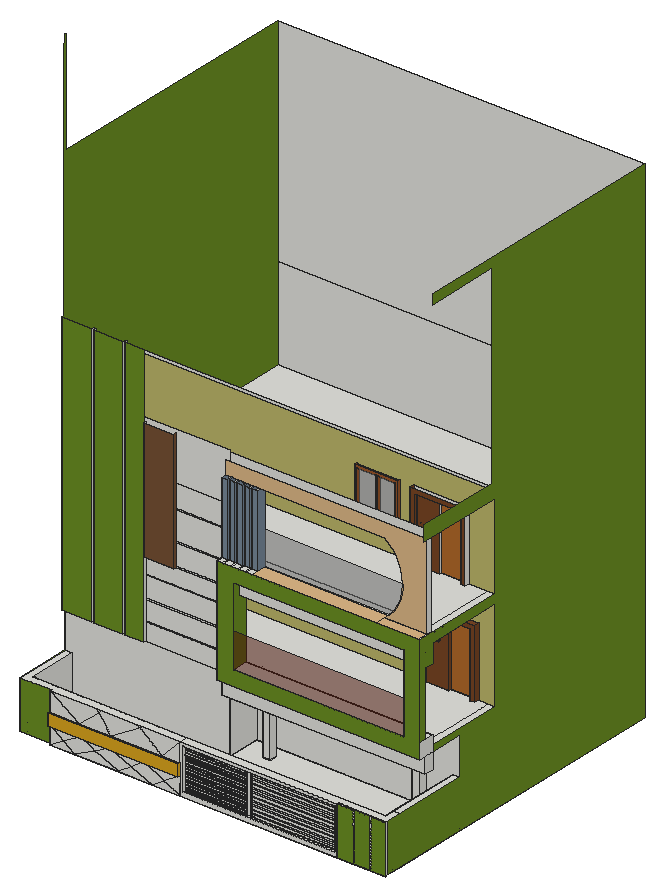
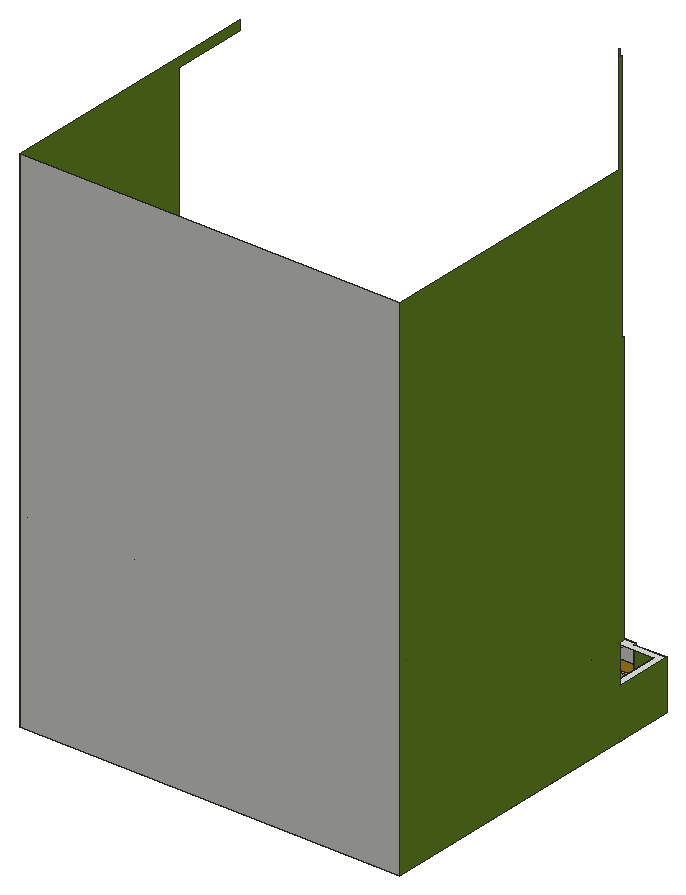
# SketchUp Ruby script. Lengths in inches.
U = 1.inch
M = Sketchup.active_model
def pt(a) = Geom::Point3d.new(a.map { |v| v * U })
def face(e, loops, mat)
  f = e.add_face(loops[0].map { |a| pt(a) })
  loops[1..].each { |l| e.add_face(l.map { |a| pt(a) }).erase! }
  f.material = f.back_material = mat if mat
  f
end
# faces: each face lists its corners as indices into pts; further lists are holes
def faces(e, pts, list, mat = nil) = list.each { |f| face(e, (f[0].is_a?(Array) ? f : [f]).map { |l| l.map { |i| pts[i] } }, mat) }
# xy, xz, yz: faces in a plane at the given z, y or x. An outline is a flat list of corners, or four numbers for a rectangle; further outlines are holes
def ring(l) = l.size == 4 ? [[l[0], l[1]], [l[2], l[1]], [l[2], l[3]], [l[0], l[3]]] : l.each_slice(2).to_a
def flat(e, list, mat, &to3) = list.each { |f| face(e, (f[0].is_a?(Array) ? f : [f]).map { |l| ring(l).map { |u, v| to3.(u, v) } }, mat) }
def xy(e, z, list, mat = nil) = flat(e, list, mat) { |x, y| [x, y, z] }
def xz(e, y, list, mat = nil) = flat(e, list, mat) { |x, z| [x, y, z] }
def yz(e, x, list, mat = nil) = flat(e, list, mat) { |y, z| [x, y, z] }
def lines(e, pts, list) = list.each { |a, b| e.add_line(pt(pts[a]), pt(pts[b])) }
# prism: a flat outline (further loops are holes) pulled along v
def prism(e, loops, v, mat = nil)
  f = face(e, loops, mat); d = Geom::Vector3d.new(v.map { |x| x * U })
  f.pushpull(f.normal.samedirection?(d) ? d.length : -d.length)
end
def box(e, o, s, mat = nil) = prism(e, [[o, [o[0] + s[0], o[1], o[2]], [o[0] + s[0], o[1] + s[1], o[2]], [o[0], o[1] + s[1], o[2]]]], [0, 0, s[2]], mat)
def at(x, y, z, deg = 0) = Geom::Transformation.translation(pt([x, y, z])) * Geom::Transformation.rotation(ORIGIN, Z_AXIS, deg.degrees)
def axes(o, x, y, z) = Geom::Transformation.new([*x, 0, *y, 0, *z, 0, *pt(o).to_a, 1])
def part(name) = M.definitions.add(name)
# library, detail: a bought-in or finely detailed component or shape, given as its bounding box
def library(name, o, s) = part(name).tap { |d| box(d.entities, o, s) }
def detail(e, o, s) = box(e.add_group.entities, o, s)
def put(e, d, t, mat = nil) = e.add_instance(d, t).tap { |i| i.material = mat if mat }
def group(e, t, mat = nil) = e.add_group.tap { |g| g.transformation = t; g.material = mat if mat }.entities
root = M.entities
M.materials.add("[0036_BurlyWood]").color = [222, 184, 135]
M.materials.add("[0045_Goldenrod]").color = [218, 165, 32]
M.materials.add("[0057_DarkKhaki]").color = [189, 183, 107]
M.materials.add("[0061_OliveDrab]").color = [107, 142, 35]
M.materials.add("[0110_LightSlateGray]").color = [119, 136, 153]
M.materials.add("[Sandstone]").color = [118, 81, 52]
M.materials.add("[Translucent Glass Dark Green]").color = [91, 24, 11]
M.materials["[Translucent Glass Dark Green]"].alpha = 0.5
M.materials.add("[Translucent Glass Gray]").color = [128, 128, 128]
M.materials["[Translucent Glass Gray]"].alpha = 0.5
M.materials.add("[Wood Bamboo]").color = [177, 105, 43]
M.materials.add("[Wood Cherry Original]").color = [152, 86, 42]
M.materials.add("[Wood Veneer 01]").color = [120, 70, 37]
xy(root,0,[[[211.33,3,417,3,417,6,480,6,480,15,471,15,471,123.9375,214.69,123.9375,214.69,79.75,9,79.75,9,15,211.33,15],[242.41,99.05,252.1,108.74],[438.16,99.05,447.85,108.74]],[40.99,3,211.33,6],[417,3,480,6],[0,6,9,15],[0,15,9,79.75],
  [471,15,480,26.9375],[471,26.9375,480,123.9375],[0,79.75,9,81.3125],[9,79.75,214.69,81.3125],[0,81.3125,9,88.75],
  [9,81.3125,9,88.75,205.69,88.75,205.69,123.9375,214.69,123.9375,214.69,81.3125],[0,88.75,9,123.9375],[9,88.75,205.69,123.9375],[242.41,99.05,252.1,108.74],[438.16,99.05,447.85,108.74],
  [0,123.9375,205.69,123.9375,205.69,132.9375,480,132.9375,480,426.3125,0,426.3125],[205.69,123.9375,205.69,129.9375,471,129.9375,471,132.9375,480,132.9375,480,123.9375],[205.69,129.9375,471,132.9375]])
xy(root,3,[[[9,15,471,15,471,123.9375,214.69,123.9375,214.69,79.75,9,79.75],[242.41,99.05,252.1,108.74],[438.16,99.05,447.85,108.74]]])
xy(root,6.12,[[215.375,3,414.15,3,414.15,6,302.66,6,302.66,15,300.97,15,300.97,6,215.375,6]])
xy(root,13.75,[[9,14.75,211.33,15],[211.33,14.75,295.89,15],[295.89,14.75,300.97,15],[302.66,14.75,471,15],[[9,15,471,15,471,123.9375,214.69,123.9375,214.69,79.75,9,79.75],[242.41,99.05,252.1,108.74],[438.16,99.05,447.85,108.74]]])
xy(root,23.125,[[40.99,0,211.33,3]],"[0045_Goldenrod]")
xy(root,38.15,[[40.99,0,211.33,3]])
xy(root,42.09,[[215.375,6,295.89,35.9375]])
xy(root,44.04,[[215.375,6,295.89,35.9375]])
xy(root,45.22,[[215.375,6,295.89,28.75]])
xy(root,47.16,[[215.375,6,295.89,28.75]])
xy(root,48.34,[[215.375,6,295.89,15]])
xy(root,50.29,[[215.375,6,295.89,15]])
xy(root,51.47,[[215.375,6,295.89,15]])
xy(root,53.41,[[215.375,6,295.89,15]])
xy(root,54.59,[[215.375,6,295.89,14.75],[215.375,14.75,295.89,15]])
xy(root,56.54,[[215.375,6,295.89,14.75],[215.375,14.75,295.89,15]])
xy(root,57.72,[[215.375,6,295.89,14.75],[215.375,14.75,295.89,15]])
xy(root,59.66,[[215.375,3,215.375,6,300.97,6,300.97,14.75,302.66,14.75,302.66,6,414.15,6,414.15,3],[215.375,6,295.89,14.75],[215.375,14.75,295.89,15],[300.97,14.75,302.66,15]])
xy(root,63,[[40.99,3,211.33,3,211.33,14.75,9,14.75,9,79.75,0,79.75,0,6,40.99,6],[211.33,3,417,3,417,6,480,6,480,26.9375,471,26.9375,471,15,211.33,15],[417,3,480,6],[9,14.75,211.33,15],[471,26.9375,480,123.9375]])
xy(root,91.22,[[214.69,67.75,480,79.75]])
xy(root,108.375,[[438.16,97.62,447.85,99.05],[438.16,99.05,447.85,108.74]])
xy(root,111.625,[[9,81.3125,214.69,123.9375]])
xy(root,112.1,[[0,73.75,0,79.75,214.69,79.75,214.69,76.75,107.35,76.75,107.35,73.75,83.22,73.75,83.22,76.75,80.57,76.75,80.57,73.75,42.34,73.75,42.34,76.75,39.7,76.75,39.7,73.75],[242.41,99.05,252.1,108.74],[252.1,99.05,253.72,108.74]])
xy(root,112.1,[[214.69,58.75,480,67.75]],"[0061_OliveDrab]")
xy(root,120,[[214.69,79.75,480,79.75,480,182.4375,471,182.4375,471,88.75,9,88.75,9,81.3125,214.69,81.3125],[9,79.75,214.69,81.3125],[9,88.75,471,88.75,471,182.4375,458.11,182.4375,458.11,176.4375,452.11,176.4375,452.11,182.4375,422.11,182.4375,422.11,179.4375,392.11,179.4375,392.11,176.4375,386.11,176.4375,386.11,182.4375,9,182.4375],[386.11,176.4375,392.11,182.4375],[452.11,176.4375,458.11,182.4375],
  [392.11,179.4375,422.11,182.4375],[9,188.4375,471,417.3125]])
xy(root,132.05,[[236.55,58.75,459.14,58.75,459.14,67.75,480,67.75,480,79.75,236.55,79.75]])
xy(root,144.9,[[283.375,179.4375,362.5625,182.4375]])
xy(root,147.9,[[286.375,179.4375,322.97,182.4375],[327.14,179.4375,359.5625,182.4375]],"[Wood Cherry Original]")
xy(root,173.57,[[395.1,177.4375,395.1,179.4375,398.85,179.4375,398.85,178.4375,405.85,178.4375,405.85,179.4375,409.6,179.4375,409.6,177.4375]],"[Wood Veneer 01]")
xy(root,174.88,[[395.1,177.4375,409.6,177.4375,409.6,179.4375,405.85,179.4375,405.85,178.4375,398.85,178.4375,398.85,179.4375,395.1,179.4375]],"[Wood Veneer 01]")
xy(root,204,[[392.11,176.4375,392.11,179.4375,422.11,179.4375,422.11,182.4375,452.11,182.4375,452.11,176.4375],[392.11,179.4375,422.11,182.4375]])
xy(root,207.33,[[286.375,179.4375,322.97,182.4375],[327.14,179.4375,359.5625,182.4375]],"[Wood Cherry Original]")
xy(root,210,[[386.11,176.4375,458.11,182.4375]],"[Wood Veneer 01]")
xy(root,210.33,[[283.375,179.4375,362.5625,182.4375]])
xy(root,212.44,[[107.35,73.75,146.78,76.75]],"[Sandstone]")
xy(root,215.25,[[236.55,67.75,480,79.75]])
xy(root,233.625,[[236.55,58.75,459.14,67.75]],"[0061_OliveDrab]")
xy(root,240,[[9,79.75,214.69,81.3125],[479.5625,79.75,480,83.125],[479.5625,83.125,480,182.4375],[9,182.4375,471,188.4375],[8.5625,188.4375,9,192.0625],
  [9,188.4375,336.04,192.0625],[336.04,188.4375,471,192.0625],[336.04,192.0625,471,417.3125]])
xy(root,240,[[214.69,79.75,214.69,81.3125,9,81.3125,9,182.4375,479.5625,182.4375,479.5625,79.75]],"[0057_DarkKhaki]")
xy(root,252,[[214.69,58.75,222.11,67.75],[222.11,58.75,224.38,79.75],[224.38,58.75,231.79,67.75],[231.79,58.75,234.07,79.75],[234.07,58.75,241.48,67.75],
  [241.48,58.75,243.75,79.75],[243.75,58.75,251.17,67.75],[251.17,58.75,253.44,79.75],[253.44,58.75,260.86,67.75],[477.8125,58.75,480,79.75],
  [214.69,67.75,222.11,79.75],[224.38,67.75,231.79,79.75],[234.07,67.75,241.48,79.75],[243.75,67.75,251.17,79.75],[253.44,67.75,260.86,79.75],
  [422.69,73.75,477.8125,79.75],[214.69,79.75,480,79.75,480,182.4375,471,182.4375,471,88.75,9,88.75,9,81.3125,214.69,81.3125],[9,79.75,214.69,81.3125],[9,88.75,471,88.75,471,182.4375,445.35,182.4375,445.35,176.4375,439.35,176.4375,439.35,182.4375,409.35,182.4375,409.35,179.4375,379.35,179.4375,379.35,176.4375,373.35,176.4375,373.35,182.4375,9,182.4375],[373.35,176.4375,379.35,182.4375],
  [439.35,176.4375,445.35,182.4375],[379.35,179.4375,409.35,182.4375],[9,188.4375,471,417.3125]])
xy(root,252,[[260.86,58.75,422.69,79.75],[422.69,58.75,477.8125,73.75]],"[0036_BurlyWood]")
xy(root,289.14,[[298.39,179.4375,354.57,182.4375]],"[Wood Cherry Original]")
xy(root,292.14,[[301.39,179.4375,326.48,182.4375],[329.2,179.4375,351.57,182.4375]],"[Wood Cherry Original]")
xz(root,0,[[40.99,23.125,211.33,38.15]],"[0045_Goldenrod]")
xz(root,3,[[40.99,0,58.6,10.14,40.99,23.125],[40.99,0,72.35,0,58.6,10.14],[72.35,0,100.12,14.13,81.16,23.125,58.6,10.14],[72.35,0,129.9,0,100.12,14.13],[129.9,0,146.75,11.24,117.79,23.125,100.12,14.13],
  [129.9,0,174.13,0,146.75,11.24],[174.13,0,190.61,10.24,164.56,23.125,146.75,11.24],[174.13,0,211.33,0,190.61,10.24],[211.33,0,211.33,23.125,190.61,10.24],[[211.33,0,417,63],[215.375,6.12,414.15,59.66]],
  [436.76,0,438.58,63],[459.14,0,460.95,63],[58.6,10.14,81.16,23.125,40.99,23.125],[190.61,10.24,211.33,23.125,164.56,23.125],[146.75,11.24,164.56,23.125,117.79,23.125],
  [100.12,14.13,117.79,23.125,81.16,23.125],[40.99,38.15,79.4,38.15,40.99,63],[79.4,38.15,104.86,59.64,102.28,63,40.99,63],[79.4,38.15,121.4,38.15,104.86,59.64],[121.4,38.15,158.25,60.54,155.04,63,108.85,63,104.86,59.64],
  [121.4,38.15,187.45,38.15,158.25,60.54],[187.45,38.15,211.33,63,162.29,63,158.25,60.54],[187.45,38.15,211.33,38.15,211.33,63],[104.86,59.64,108.85,63,102.28,63],[158.25,60.54,162.29,63,155.04,63]])
xz(root,3,[[417,0,436.76,63],[438.58,0,459.14,63],[460.95,0,480,63]],"[0061_OliveDrab]")
xz(root,6,[[40.99,0,211.33,3],[417,0,480,63],[302.66,0.71,414.15,3.97],[215.375,1.47,295.89,3.41],[40.99,3,211.33,13.75],
  [215.375,4.59,295.89,6.12],[302.66,5.77,414.15,6.12],[215.375,6.12,295.89,6.54],[295.89,6.12,300.97,59.66],[302.66,6.12,414.15,9.04],
  [215.375,6.54,295.89,7.72],[215.375,7.72,295.89,9.66],[302.66,9.04,414.15,10.84],[215.375,9.66,295.89,10.84],[215.375,10.84,295.89,12.79],
  [302.66,10.84,414.15,14.1],[215.375,12.79,295.89,13.97],[215.375,13.97,295.89,15.91],[302.66,14.1,414.15,15.9],[302.66,15.9,414.15,19.16],
  [215.375,15.91,295.89,17.09],[215.375,17.09,295.89,19.04],[215.375,19.04,295.89,20.22],[302.66,19.16,414.15,20.96],[215.375,20.22,295.89,22.16],
  [302.66,20.96,414.15,24.22],[215.375,22.16,295.89,23.34],[215.375,23.34,295.89,25.29],[302.66,24.22,414.15,26.02],[215.375,25.29,295.89,26.47],
  [302.66,26.02,414.15,29.29],[215.375,26.47,295.89,28.41],[215.375,28.41,295.89,29.59],[302.66,29.29,414.15,31.09],[215.375,29.59,295.89,31.54],
  [302.66,31.09,414.15,34.35],[215.375,31.54,295.89,32.72],[215.375,32.72,295.89,34.66],[302.66,34.35,414.15,36.15],[215.375,34.66,295.89,35.84],
  [215.375,35.84,295.89,37.79],[302.66,36.15,414.15,39.41],[215.375,37.79,295.89,38.97],[215.375,38.97,295.89,40.91],[302.66,39.41,414.15,41.21],
  [215.375,40.91,295.89,42.09],[302.66,41.21,414.15,44.47],[215.375,42.09,295.89,44.04],[215.375,44.04,295.89,45.22],[302.66,44.47,414.15,46.27],
  [215.375,45.22,295.89,47.16],[302.66,46.27,414.15,49.54],[215.375,47.16,295.89,48.34],[215.375,48.34,295.89,50.29],[302.66,49.54,414.15,51.34],
  [215.375,50.29,295.89,51.47],[302.66,51.34,414.15,54.6],[215.375,51.47,295.89,53.41],[215.375,53.41,295.89,54.59],[215.375,54.59,295.89,56.54],
  [302.66,54.6,414.15,56.4],[302.66,56.4,414.15,59.66],[215.375,56.54,295.89,57.72],[215.375,57.72,295.89,59.66]])
xz(root,6,[[0,0,40.99,63]],"[0061_OliveDrab]")
xz(root,15,[[9,3,9,13.75,300.97,13.75,300.97,6.12,302.66,6.12,302.66,13.75,471,13.75,471,3],[300.97,6.12,302.66,13.75]])
xz(root,28.75,[[215.375,45.22,295.89,47.16]])
xz(root,35.9375,[[215.375,42.09,295.89,44.04]])
xz(root,58.75,[[214.69,112.1,480,112.1,480,132.05,236.55,132.05,236.55,233.625,459.14,233.625,459.14,132.05,480,132.05,480,252,214.69,252]],"[0061_OliveDrab]")
xz(root,58.75,[[236.55,132.05,459.14,177.7]],"[Translucent Glass Dark Green]")
xz(root,67.75,[[214.69,91.22,480,112.1],[459.14,132.05,480,215.25],[236.55,215.25,459.14,233.625]])
xz(root,67.75,[[214.69,252,222.11,345.55],[224.38,252,231.79,345.55],[234.07,252,241.48,345.55],[243.75,252,251.17,345.55],[253.44,252,260.86,345.55]],"[0110_LightSlateGray]")
xz(root,73.75,[[422.69,252,477.8125,252,477.8125,363.8125,214.69,363.8125,214.69,345.55,422.69,345.55,429.47,339.59,435.25,332.66,439.9,324.92,443.3,316.56,445.37,307.78,446.07,298.78,445.37,289.78,443.3,280.99,439.9,272.63,435.25,264.89,429.47,257.96]],"[0036_BurlyWood]")
xz(root,73.75,[[0,112.1,39.7,455],[42.34,112.1,80.57,455],[83.22,112.1,107.35,455]],"[0061_OliveDrab]")
xz(root,73.75,[[107.35,212.44,146.78,369.44]],"[Sandstone]")
xz(root,76.75,[[39.7,112.1,42.34,455],[80.57,112.1,83.22,455],[107.35,112.1,214.69,134.76],[107.35,134.76,214.69,136.29],[107.35,136.29,214.69,161.07],
  [107.35,161.07,214.69,162.61],[107.35,162.61,214.69,190.01],[107.35,190.01,214.69,191.54],[107.35,191.54,214.69,191.54,214.69,212.26,146.78,212.26,146.78,212.44,107.35,212.44],[146.78,212.26,214.69,214.11],
  [107.35,212.44,146.78,366.59],[146.78,214.11,214.69,241.33],[146.78,241.33,214.69,243.18],[146.78,243.18,214.69,279.89],[146.78,279.89,214.69,281.74],
  [146.78,281.74,214.69,310.89]])
xz(root,79.75,[[9,0,214.69,3],[9,3,214.69,13.75],[9,13.75,214.69,13.75,214.69,112.1,0,112.1,0,63,9,63],[214.69,91.22,480,112.1],[214.69,112.1,480,120],
  [9,120,214.69,240],[214.69,120,214.69,215.25,236.55,215.25,236.55,132.05,480,132.05,480,120],[214.69,215.25,480,240],[9,252,214.69,372],[446.07,252,446.07,296.15,445.86,296.15,446.07,298.78,445.37,307.78,443.3,316.56,439.9,324.92,435.25,332.66,429.47,339.59,422.69,345.55,214.69,345.55,214.69,370.625,477.8125,370.625,477.8125,252],
  [422.69,252,429.47,257.96,435.25,264.89,439.9,272.63,443.3,280.99,445.37,289.78,445.86,296.15,446.07,296.15,446.07,252]])
xz(root,79.75,[[214.69,252,222.11,296.15],[222.11,252,224.38,296.15],[224.38,252,231.79,296.15],[231.79,252,234.07,296.15],[234.07,252,241.48,296.15],
  [241.48,252,243.75,296.15],[243.75,252,251.17,296.15],[251.17,252,253.44,296.15],[253.44,252,260.86,296.15],[260.86,252,260.86,296.15,445.86,296.15,445.37,289.78,443.3,280.99,439.9,272.63,435.25,264.89,429.47,257.96,422.69,252]],"[Translucent Glass Gray]")
xz(root,81.3125,[[9,0,214.69,111.625],[9,111.625,214.69,112.1]])
xz(root,99.05,[[242.41,0,252.1,3],[438.16,0,447.85,3],[242.41,3,252.1,13.75],[438.16,3,447.85,13.75],[242.41,13.75,252.1,112.1],
  [438.16,13.75,447.85,108.375]])
xz(root,108.74,[[242.41,0,252.1,3],[438.16,0,447.85,3],[242.41,3,252.1,13.75],[438.16,3,447.85,13.75],[242.41,13.75,252.1,112.1],
  [438.16,13.75,447.85,77.75],[438.16,77.75,447.85,108.375]])
xz(root,123.9375,[[9,0,214.69,111.625],[214.69,0,471,3],[214.69,3,471,13.75],[214.69,13.75,471,13.75,471,63,480,63,480,112.1,9,112.1,9,111.625,214.69,111.625]])
xz(root,176.4375,[[386.11,120,392.11,120,392.11,204,452.11,204,452.11,120,458.11,120,458.11,210,386.11,210],[373.35,252,379.35,252,379.35,336,439.35,336,439.35,252,445.35,252,445.35,342,373.35,342]],"[Wood Veneer 01]")
xz(root,177.4375,[[395.1,173.57,409.6,174.88]],"[Wood Veneer 01]")
xz(root,178.4375,[[398.85,173.57,405.85,174.88]])
xz(root,179.4375,[[[283.375,144.9,362.5625,210.33],[286.375,147.9,322.97,207.33],[327.14,147.9,359.5625,207.33]],[[298.39,289.14,354.57,341.33],[301.39,292.14,326.48,338.33],[329.2,292.14,351.57,338.33]]],"[Wood Cherry Original]")
xz(root,179.4375,[[[392.11,120,422.11,204],[395.1,173.57,398.85,174.88],[405.85,173.57,409.6,174.88]],[[379.35,252,409.35,336],[383.79,302.01,386.62,303.76],[395.22,302.01,398.06,303.76]]],"[Wood Veneer 01]")
xz(root,182.4375,[[386.11,114,458.11,120],[392.11,120,422.11,204],[[283.375,144.9,362.5625,210.33],[286.375,147.9,322.97,207.33],[327.14,147.9,359.5625,207.33]],[373.35,246,445.35,252],[373.35,252,373.35,342,445.35,342,445.35,252,439.35,252,439.35,336,379.35,336,379.35,252],
  [379.35,252,409.35,336],[[298.39,289.14,354.57,341.33],[301.39,292.14,326.48,338.33],[329.2,292.14,351.57,338.33]]])
xz(root,182.4375,[[[9,120,386.11,120,386.11,210,458.11,210,458.11,120,480,120,480,240,9,240],[283.375,144.9,362.5625,210.33]],[[9,252,373.35,252,373.35,342,445.35,342,445.35,252,480,252,480,363.8125,477.8125,363.8125,477.8125,372,9,372],[298.39,289.14,354.57,341.33]]],"[0057_DarkKhaki]")
xz(root,182.4375,[[286.375,147.9,322.97,207.33],[327.14,147.9,359.5625,207.33],[301.39,292.14,326.48,338.33],[329.2,292.14,351.57,338.33]],"[Translucent Glass Gray]")
xz(root,182.4375,[[422.11,120,452.11,204],[409.35,252,439.35,336]],"[Wood Bamboo]")
xz(root,188.4375,[[9,120,471,240],[9,252,471,372]])
xz(root,417.3125,[[9,120,471,240],[9,252,471,372]])
xz(root,426.3125,[[0,0,480,648]])
yz(root,0,[[6,0,6,63,79.75,63,79.75,112.1,73.75,112.1,73.75,455,76.75,455,76.75,774.38,79.75,774.38,79.75,784.0625,81.3125,784.0625,81.3125,648,426.3125,648,426.3125,0]],"[0061_OliveDrab]")
yz(root,9,[[15,0,79.75,3],[81.3125,0,123.9375,111.625],[15,3,79.75,3.75],[15,3.75,79.75,3.9375],[15,3.9375,79.75,13.75],
  [14.75,13.75,15,63],[15,13.75,79.75,63],[81.3125,111.625,123.9375,112.5],[79.75,120,81.3125,240],[81.3125,120,88.75,240],
  [88.75,120,182.4375,240],[188.4375,120,417.3125,240],[79.75,252,81.3125,372],[81.3125,252,88.75,372],[88.75,252,182.4375,372]])
yz(root,39.7,[[73.75,112.1,76.75,455]])
yz(root,40.99,[[3,0,3,23.125,0,23.125,0,38.15,3,38.15,3,63,6,63,6,0]],"[0045_Goldenrod]")
yz(root,42.34,[[73.75,112.1,76.75,455]])
yz(root,80.57,[[73.75,112.1,76.75,455]])
yz(root,83.22,[[73.75,112.1,76.75,455]])
yz(root,107.35,[[73.75,112.1,76.75,212.44],[73.75,212.44,76.75,369.44]])
yz(root,146.78,[[73.75,212.44,76.75,369.44]],"[Sandstone]")
yz(root,211.33,[[3,0,6,3],[6,0,26.9375,3],[3,3,6,13.75]])
yz(root,211.33,[[0,23.125,3,38.15]],"[0045_Goldenrod]")
yz(root,214.69,[[79.75,0,81.3125,3],[81.3125,0,123.9375,3],[79.75,3,81.3125,13.75],[81.3125,3,123.9375,13.75],[79.75,13.75,81.3125,112.1],
  [81.3125,13.75,123.9375,111.625],[76.75,91.22,79.75,112.1],[76.75,112.1,79.75,120],[79.75,112.1,81.3125,120],[76.75,120,76.75,213.87,79.75,215.25,79.75,120],
  [76.75,213.87,76.75,252,79.75,252,79.75,215.25],[79.75,240,81.3125,252],[76.75,252,79.75,345.55]])
yz(root,214.69,[[67.75,91.22,67.75,112.1,58.75,112.1,58.75,252,76.75,252,76.75,91.22]],"[0061_OliveDrab]")
yz(root,214.69,[[67.75,252,76.75,345.55]],"[0110_LightSlateGray]")
yz(root,215.375,[[3,6.12,6,59.66],[6,42.09,35.9375,44.04],[6,45.22,28.75,47.16],[6,48.34,15,50.29],[6,51.47,15,53.41],
  [6,54.59,14.75,56.54],[14.75,54.59,15,56.54],[6,57.72,14.75,59.66],[14.75,57.72,15,59.66]])
yz(root,222.11,[[67.75,252,79.75,345.55]],"[0110_LightSlateGray]")
yz(root,224.38,[[76.75,252,79.75,345.55]])
yz(root,224.38,[[67.75,252,76.75,345.55]],"[0110_LightSlateGray]")
yz(root,231.79,[[67.75,252,79.75,345.55]],"[0110_LightSlateGray]")
yz(root,234.07,[[76.75,252,79.75,345.55]])
yz(root,234.07,[[67.75,252,76.75,345.55]],"[0110_LightSlateGray]")
yz(root,236.55,[[58.75,132.05,79.75,132.05,79.75,215.25,67.75,215.25,67.75,233.625,58.75,233.625]],"[0061_OliveDrab]")
yz(root,241.48,[[67.75,252,79.75,345.55]],"[0110_LightSlateGray]")
yz(root,242.41,[[99.05,0,108.74,3],[99.05,3,108.74,13.75],[99.05,13.75,108.74,112.1]])
yz(root,243.75,[[76.75,252,79.75,345.55]])
yz(root,243.75,[[67.75,252,76.75,345.55]],"[0110_LightSlateGray]")
yz(root,251.17,[[67.75,252,79.75,345.55]],"[0110_LightSlateGray]")
yz(root,252.1,[[99.05,0,108.74,3],[99.05,3,108.74,13.75],[99.05,13.75,108.74,112.1]])
yz(root,253.44,[[76.75,252,79.75,345.55]])
yz(root,253.44,[[67.75,252,76.75,345.55]],"[0110_LightSlateGray]")
yz(root,260.86,[[67.75,252,79.75,345.55]],"[0110_LightSlateGray]")
yz(root,283.375,[[179.4375,144.9,182.4375,210.33]])
yz(root,286.375,[[179.4375,147.9,182.4375,207.33]],"[Wood Cherry Original]")
yz(root,295.89,[[6,6.12,6,42.09,14.75,42.09,14.75,13.75,15,13.75,15,6.12],[14.75,13.75,15,42.09],[6,42.09,14.75,44.04],[14.75,42.09,15,44.04],[15,42.09,35.9375,44.04],
  [6,44.04,14.75,45.22],[14.75,44.04,15,45.22],[6,45.22,14.75,47.16],[14.75,45.22,15,47.16],[15,45.22,28.75,47.16],
  [6,47.16,14.75,48.34],[14.75,47.16,15,48.34],[6,48.34,14.75,50.29],[14.75,48.34,15,50.29],[6,50.29,14.75,51.47],
  [14.75,50.29,15,51.47],[6,51.47,14.75,53.41],[14.75,51.47,15,53.41],[6,53.41,14.75,54.59],[14.75,53.41,15,54.59],
  [6,54.59,14.75,56.54],[14.75,54.59,15,56.54],[6,56.54,14.75,57.72],[14.75,56.54,15,57.72],[6,57.72,14.75,59.66],
  [14.75,57.72,15,59.66]])
yz(root,298.39,[[179.4375,289.14,182.4375,341.33]],"[Wood Cherry Original]")
yz(root,300.97,[[6,6.12,15,6.12,15,13.75,14.75,13.75,14.75,59.66,6,59.66],[14.75,13.75,15,59.66]])
yz(root,301.39,[[179.4375,292.14,182.4375,338.33]],"[Wood Cherry Original]")
yz(root,302.66,[[6,6.12,6,59.66,14.75,59.66,14.75,13.75,15,13.75,15,6.12],[14.75,13.75,15,59.66]])
yz(root,322.97,[[179.4375,147.9,182.4375,207.33]],"[Wood Cherry Original]")
yz(root,326.48,[[179.4375,292.14,182.4375,338.33]],"[Wood Cherry Original]")
yz(root,327.14,[[179.4375,147.9,182.4375,207.33]],"[Wood Cherry Original]")
yz(root,329.2,[[179.4375,292.14,182.4375,338.33]],"[Wood Cherry Original]")
yz(root,351.57,[[179.4375,292.14,182.4375,338.33]],"[Wood Cherry Original]")
yz(root,354.57,[[179.4375,289.14,182.4375,341.33]],"[Wood Cherry Original]")
yz(root,359.5625,[[179.4375,147.9,182.4375,207.33]],"[Wood Cherry Original]")
yz(root,362.5625,[[179.4375,144.9,182.4375,210.33]],"[Wood Cherry Original]")
yz(root,373.35,[[176.4375,252,182.4375,342]],"[Wood Veneer 01]")
yz(root,379.35,[[179.4375,252,182.4375,336]])
yz(root,379.35,[[176.4375,252,179.4375,336]],"[Wood Veneer 01]")
yz(root,386.11,[[176.4375,120,182.4375,210]],"[Wood Veneer 01]")
yz(root,392.11,[[179.4375,120,182.4375,204]])
yz(root,392.11,[[176.4375,120,179.4375,204]],"[Wood Veneer 01]")
yz(root,395.1,[[177.4375,173.57,179.4375,174.88]],"[Wood Veneer 01]")
yz(root,398.85,[[178.4375,173.57,179.4375,174.88]],"[Wood Veneer 01]")
yz(root,405.85,[[178.4375,173.57,179.4375,174.88]],"[Wood Veneer 01]")
yz(root,409.35,[[179.4375,252,182.4375,336]])
yz(root,409.6,[[177.4375,173.57,179.4375,174.88]],"[Wood Veneer 01]")
yz(root,414.15,[[3,6.12,6,59.66]])
yz(root,417,[[3,0,6,63]])
yz(root,422.11,[[179.4375,120,182.4375,204]],"[Wood Veneer 01]")
yz(root,438.16,[[99.05,0,108.74,3],[99.05,3,108.74,13.75],[99.05,13.75,108.74,108.375]])
yz(root,439.35,[[176.4375,252,182.4375,336]],"[Wood Veneer 01]")
yz(root,445.35,[[176.4375,252,182.4375,342]])
yz(root,447.85,[[99.05,0,108.74,3],[99.05,3,108.74,13.75],[99.05,13.75,108.74,108.375]])
yz(root,452.11,[[176.4375,120,182.4375,204]],"[Wood Veneer 01]")
yz(root,458.11,[[176.4375,120,182.4375,210]],"[Wood Veneer 01]")
yz(root,459.14,[[58.75,132.05,67.75,233.625]],"[0061_OliveDrab]")
yz(root,471,[[15,0,123.9375,3],[15,3,123.9375,13.75],[14.75,13.75,15,63],[15,13.75,123.9375,63],[188.4375,120,417.3125,240],
  [188.4375,252,417.3125,372]])
yz(root,477.8125,[[73.75,252,79.75,363.8125]])
yz(root,480,[[3,0,6,63],[67.75,91.22,79.75,112.1],[58.75,112.1,79.75,132.05]])
yz(root,480,[[6,0,426.3125,0,426.3125,648,79.75,648,79.75,636,176.4375,636,176.4375,384,65.75,384,65.75,363.8125,182.4375,363.8125,182.4375,252,58.75,252,58.75,132.05,67.75,132.05,67.75,215.25,79.75,215.25,79.75,240,182.4375,240,182.4375,120,79.75,120,79.75,112.1,123.9375,112.1,123.9375,63,6,63]],"[0061_OliveDrab]")
p = [[429.47,79.75,257.96],[422.69,79.75,252],[422.69,73.75,252],[429.47,73.75,257.96],[435.25,79.75,264.89],[435.25,73.75,264.89],
  [439.9,79.75,272.63],[439.9,73.75,272.63],[443.3,79.75,280.99],[443.3,73.75,280.99],[445.37,79.75,289.78],[445.37,73.75,289.78],
  [446.07,79.75,298.78],[445.86,79.75,296.15],[446.07,73.75,298.78],[9,417.3125,0],[9,129.9375,0],[471,129.9375,0],
  [471,129.9375,120],[471,417.3125,0],[471,417.3125,120],[9,129.9375,120],[9,417.3125,120],[336.04,417.3125,240],
  [336.04,417.3125,252],[471,417.3125,240],[471,426.3125,240],[336.04,426.3125,240],[9,417.3125,240],[0,417.3125,240],
  [9,76.75,252],[9,79.75,252],[9,79.75,240],[9,76.75,240],[9,79.75,120],[9,76.75,120],
  [480,67.75,233.625],[459.14,67.75,233.625],[236.55,67.75,215.25],[214.69,67.75,215.25],[9,81.3125,111.625],[0,81.3125,111.625],
  [9,123.9375,111.625],[0,123.9375,111.625],[9,123.9375,112.5],[0,123.9375,112.5],[9,81.3125,112.5],[0,81.3125,112.5],
  [9,123.9375,112.1],[0,123.9375,112.1],[447.85,108.74,108.375],[447.85,108.74,120],[447.85,99.05,108.375],[447.85,99.05,120],
  [438.16,108.74,108.375],[438.16,108.74,120],[242.41,99.05,112.1],[242.41,99.05,120],[438.16,97.62,108.375],[438.16,97.62,120],
  [447.85,97.62,108.375],[447.85,97.62,120],[471,132.9375,0],[205.69,129.9375,0],[9,15,3],[9,6,3],
  [471,15,3],[471,6,3],[0,15,3],[9,79.75,3.9375],[0,79.75,3.9375],[9,15,3.75],
  [0,15,3.75],[9,79.75,3.75],[0,79.75,3.75],[211.33,26.9375,13.75],[211.33,26.9375,3],[211.33,6,13.75],
  [211.33,14.75,13.75],[480,15,3],[471,123.9375,3],[480,123.9375,3],[215.375,6,0.29],[295.89,6,0.29],
  [9,14.75,13.75],[9,6,13.75],[471,14.75,13.75],[471,6,13.75]]
faces(root,p,[[0,1,2,3],[4,0,3,5],[6,4,5,7],[8,6,7,9],[10,8,9,11],[12,13,10,11,14]],"[0036_BurlyWood]")
lines(root,p,[[15,16],[17,18],[19,20],[16,21],[15,22],[23,24],[25,26],[23,27],[28,29],[30,31],[32,33],[34,35],
  [36,37],[38,39],[40,41],[42,43],[44,45],[46,47],[48,49],[50,51],[52,53],[54,55],[56,57],[58,59],
  [60,61],[62,19],[63,16],[64,65],[66,67],[64,68],[69,70],[71,72],[73,74],[75,76],[77,78],[66,79],
  [80,81],[82,83],[84,85],[86,87]])
